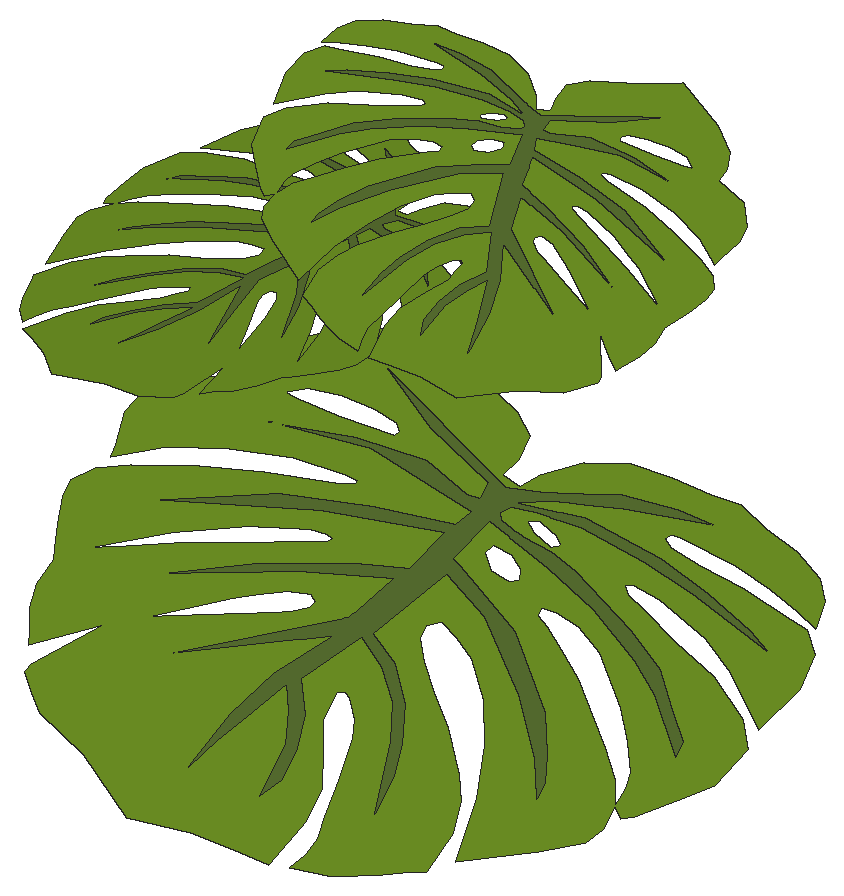
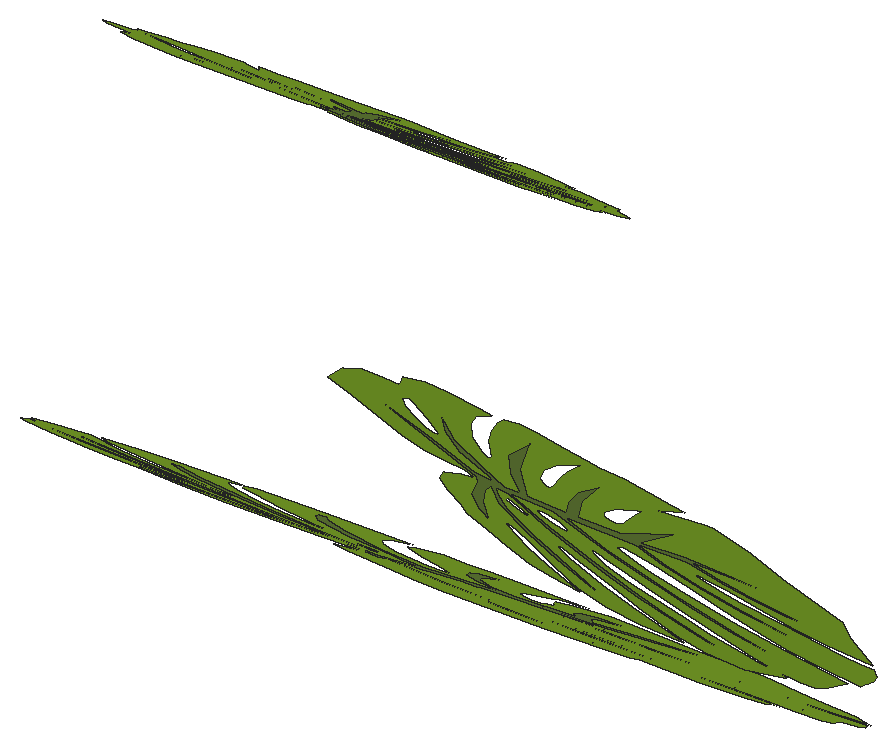
# SketchUp Ruby script. Lengths in inches.
U = 1.inch
M = Sketchup.active_model
def pt(a) = Geom::Point3d.new(a.map { |v| v * U })
def face(e, loops, mat)
  f = e.add_face(loops[0].map { |a| pt(a) })
  loops[1..].each { |l| e.add_face(l.map { |a| pt(a) }).erase! }
  f.material = f.back_material = mat if mat
  f
end
# faces: each face lists its corners as indices into pts; further lists are holes
def faces(e, pts, list, mat = nil) = list.each { |f| face(e, (f[0].is_a?(Array) ? f : [f]).map { |l| l.map { |i| pts[i] } }, mat) }
# xy, xz, yz: faces in a plane at the given z, y or x. An outline is a flat list of corners, or four numbers for a rectangle; further outlines are holes
def ring(l) = l.size == 4 ? [[l[0], l[1]], [l[2], l[1]], [l[2], l[3]], [l[0], l[3]]] : l.each_slice(2).to_a
def flat(e, list, mat, &to3) = list.each { |f| face(e, (f[0].is_a?(Array) ? f : [f]).map { |l| ring(l).map { |u, v| to3.(u, v) } }, mat) }
def xy(e, z, list, mat = nil) = flat(e, list, mat) { |x, y| [x, y, z] }
def xz(e, y, list, mat = nil) = flat(e, list, mat) { |x, z| [x, y, z] }
def yz(e, x, list, mat = nil) = flat(e, list, mat) { |y, z| [x, y, z] }
def lines(e, pts, list) = list.each { |a, b| e.add_line(pt(pts[a]), pt(pts[b])) }
# prism: a flat outline (further loops are holes) pulled along v
def prism(e, loops, v, mat = nil)
  f = face(e, loops, mat); d = Geom::Vector3d.new(v.map { |x| x * U })
  f.pushpull(f.normal.samedirection?(d) ? d.length : -d.length)
end
def box(e, o, s, mat = nil) = prism(e, [[o, [o[0] + s[0], o[1], o[2]], [o[0] + s[0], o[1] + s[1], o[2]], [o[0], o[1] + s[1], o[2]]]], [0, 0, s[2]], mat)
def at(x, y, z, deg = 0) = Geom::Transformation.translation(pt([x, y, z])) * Geom::Transformation.rotation(ORIGIN, Z_AXIS, deg.degrees)
def axes(o, x, y, z) = Geom::Transformation.new([*x, 0, *y, 0, *z, 0, *pt(o).to_a, 1])
def part(name) = M.definitions.add(name)
# library, detail: a bought-in or finely detailed component or shape, given as its bounding box
def library(name, o, s) = part(name).tap { |d| box(d.entities, o, s) }
def detail(e, o, s) = box(e.add_group.entities, o, s)
def put(e, d, t, mat = nil) = e.add_instance(d, t).tap { |i| i.material = mat if mat }
def group(e, t, mat = nil) = e.add_group.tap { |g| g.transformation = t; g.material = mat if mat }.entities
root = M.entities
M.materials.add("[0059_DarkOliveGreen]").color = [85, 107, 47]
M.materials.add("[0061_OliveDrab]").color = [107, 142, 35]
p = [[188.129,149.193,18.099],[188.867,149.058,18.014],[189.298,149.585,18.348],[190.36,150.31,18.808],[191.818,150.755,19.091],[193.373,150.829,19.137],
  [194.933,150.763,19.096],[196.031,150.815,19.129],[197.325,150.449,18.897],[198.752,150.179,18.725],[199.994,149.73,18.44],[200.614,149.188,18.096],
  [200.915,148.399,17.595],[199.983,148.646,17.752],[198.718,148.953,17.947],[197.142,149.21,18.11],[194.901,149.364,18.208],[194.528,149.346,18.197],
  [194.422,149.173,18.087],[194.792,149.025,17.992],[196.049,148.844,17.878],[197.794,148.7,17.786],[199.955,148.392,17.591],[200.649,148.277,17.518],
  [201.39,147.705,17.155],[201.656,146.671,16.499],[201.213,145.244,15.593],[199.186,146.416,16.337],[197.722,147.038,16.732],[195.507,147.571,17.07],
  [194.395,147.678,17.138],[194.138,147.574,17.072],[194.419,147.371,16.943],[195.175,147.16,16.809],[196.834,146.638,16.477],[198.753,146.128,16.154],
  [200.526,145.311,15.636],[201.296,144.606,15.188],[201.01,143.35,14.391],[200.17,142.585,13.905],[199.179,141.75,13.375],[198.796,141.571,13.262],
  [198.359,141.816,13.417],[198.34,142.391,13.782],[198.164,142.833,14.063],[197.452,143.604,14.552],[196.535,144.398,15.056],[194.732,145.61,15.825],
  [193.58,146.062,16.112],[192.594,146.201,16.2],[192.047,146.175,16.184],[192.087,145.93,16.028],[192.577,145.743,15.91],[193.472,145.3,15.629],
  [194.609,144.73,15.267],[195.942,143.84,14.702],[196.825,143.226,14.3125],[197.843,142.494,13.848],[198.477,141.088,12.955],[198.226,140.6,12.646],
  [196.938,139.896,12.199],[194.606,138.8,11.503],[193.981,140.617,12.657],[193.129,142.056,13.57],[192.137,143.23,14.315],[190.932,144.16,14.905],
  [190.019,144.561,15.159],[189.248,144.796,15.308],[188.854,144.543,15.148],[188.918,144.151,14.899],[189.522,143.599,14.549],[190.445,142.922,14.119],
  [191.601,142.158,13.635],[192.928,141.049,12.931],[193.535,140.393,12.514],[193.953,139.485,11.938],[193.917,138.258,11.159],[193.201,137.991,10.99],
  [192.644,137.733,10.826],[191.891,137.439,10.64],[190.959,137.164,10.465],[189.647,136.965,10.339],[189.848,137.459,10.653],[189.903,138.002,10.997],
  [189.65,138.637,11.4],[189.357,139.697,12.073],[188.928,140.921,12.85],[188.577,141.433,13.174],[188.004,141.944,13.499],[187.687,142.048,13.564],
  [187.478,141.93,13.49],[187.541,141.541,13.243],[187.618,141.066,12.941],[188.221,140.343,12.483],[189.007,139.283,11.81],[189.164,138.318,11.197],
  [188.938,136.839,10.259],[187.796,136.88,10.285],[185.892,136.872,10.28],[183.578,136.626,10.124],[180.962,137.808,10.874],[178.746,138.425,11.265],
  [178.105,138.881,11.555],[177.463,139.337,11.844],[177.507,139.613,12.019],[178.941,141.333,13.111],[177.775,140.577,12.631],[177.012,140.075,12.3125],
  [176.793,140.418,12.53],[176.307,141.026,12.916],[176.024,141.733,13.365],[176.039,142.501,13.852],[175.829,142.83,14.061],[175.425,143.481,14.474],
  [175.025,144.212,14.938],[174.931,144.734,15.269],[175.457,145.287,15.62],[176.472,145.703,15.884],[178.588,146.355,16.298],[180.695,146.882,16.633],
  [183.311,147.344,16.926],[183.782,147.484,17.014],[183.766,147.585,17.079],[183.287,147.633,17.109],[181.351,147.541,17.051],[179.186,147.123,16.786],
  [177.216,146.524,16.405],[175.678,145.718,15.894],[175.621,146.07,16.117],[175.211,146.999,16.707],[175.365,147.705,17.155],[176.295,148.579,17.709],
  [178.131,149.062,18.016],[178.046,149.587,18.349],[178.464,150.324,18.817],[179.9,151.18,19.36],[182.852,152.287,20.0625],[183.878,151.906,19.821],
  [185.497,151.464,19.541],[187.227,150.962,19.222],[188.163,150.469,18.909],[188.28,149.748,18.451],[186.321,144.017,14.814],[181.293,141.142,12.99],
  [186.24,143.358,14.396],[185.177,141.829,13.426],[184.672,140.327,12.472],[184.468,138.685,11.431],[184.456,138.537,11.336],[184.807,139.528,11.965],
  [185.147,140.273,12.438],[185.754,141.671,13.326],[186.359,140.997,12.898],[186.98,140.081,12.316],[187.232,138.529,11.331],[187.557,139.162,11.733],
  [187.407,140.089,12.321],[186.938,141.057,12.936],[186.087,141.953,13.504],[187.106,143.621,14.563],[188.335,143.066,14.211],[189.379,142.273,13.708],
  [190.165,141.23,13.045],[191.141,139.208,11.762],[190.956,140.348,12.486],[190.562,141.259,13.064],[189.802,142.331,13.745],[188.691,143.264,14.336],
  [187.386,143.8,14.676],[188.417,146.099,16.136],[190.482,145.372,15.674],[193.14,143.709,14.619],[194.924,142.243,13.688],[195.809,141.238,13.05],
  [195.735,141.694,13.34],[195.208,142.46,13.826],[194.277,143.523,14.501],[191.711,145.279,15.615],[190.098,145.909,16.015],[188.343,146.554,16.424],
  [188.687,147.865,17.256],[191.387,147.275,16.882],[193.696,146.646,16.483],[195.989,145.748,15.913],[197.288,145.093,15.497],[199.197,143.709,14.619],
  [199.125,144.153,14.901],[198.127,144.865,15.353],[196.931,145.765,15.924],[195.251,146.495,16.387],[192.3,147.451,16.993],[191.169,147.717,17.162],
  [189.991,147.814,17.224],[189.006,148.021,17.355],[188.827,148.205,17.472],[189.074,148.436,17.619],[189.921,148.55,17.691],[191.639,148.63,17.742],
  [194.227,148.373,17.579],[196.396,148.036,17.365],[199.833,147.347,16.928],[198.913,147.683,17.141],[196.86,148.225,17.485],[194.69,148.65,17.754],
  [191.522,148.919,17.925],[189.167,148.628,17.741],[190.269,149.024,17.992],[192.528,149.564,18.335],[195.591,150.03,18.63],[194.197,150.061,18.65],
  [192.205,149.877,18.534],[189.719,149.184,18.094],[188.455,148.922,17.927],[182.115,150.875,19.167],[184.903,149.66,18.396],[187.812,148.843,17.877],
  [187.888,148.371,17.578],[187.406,148.349,17.563],[185.477,148.816,17.86],[182.827,148.691,17.781],[179.841,148.194,17.465],[183.537,148.534,17.681],
  [186.02,148.188,17.462],[187.893,147.932,17.299],[187.683,147.459,16.999],[184.743,147.095,16.768],[181.598,146.492,16.385],[177.819,145.024,15.453],
  [183.264,146.4375,16.351],[187.487,147.13,16.79],[187.168,145.88,15.996],[185.391,145.463,15.732],[182.37,144.471,15.102],[179.481,143.175,14.28],
  [183.852,144.676,15.232],[186.868,145.42,15.705],[181.318,145.322,15.642],[179.931,144.754,15.282],[179.158,144.4375,15.081],[176.818,143.148,14.263],
  [177.739,143.491,14.48],[179.664,144.237,14.954],[181.6,144.884,15.365],[183.364,145.465,15.733],[184.099,145.711,15.889],[184.188,145.851,15.978],
  [183.917,145.913,16.018],[183.288,145.862,15.985],[183.102,143.689,14.606],[182.702,143.504,14.489],[182.317,143.327,14.376],[180.069,141.98,13.522],
  [181.913,142.642,13.942],[183.894,143.363,14.399],[184.397,143.538,14.51],[184.888,143.847,14.706],[184.964,144.066,14.845],[184.652,144.207,14.935],
  [183.888,144.05,14.835],[182.142,149.616,18.368],[181.478,149.63,18.376],[180.354,149.474,18.277],[179.71,149.129,18.059],[180.136,149.073,18.023],
  [181.896,149.053,18.011],[184.003,149.103,18.042],[184.069,149.259,18.141],[183.778,149.465,18.272],[182.806,149.603,18.359],[189.158,147.003,16.709],
  [189.695,146.619,16.466],[190.486,146.503,16.392],[190.797,146.639,16.478],[190.6,146.975,16.692],[190.022,147.242,16.861],[189.288,147.297,16.896],
  [190.742,148.251,17.501],[190.201,148.378,17.582],[189.807,148.252,17.502],[190.259,148.022,17.356],[191.078,147.823,17.23],[191.374,147.974,17.325],
  [190.964,148.199,17.468],[186.512,151.899,25.1],[187.3,151.802,25.26],[187.777,150.495,24.796],[187.751,149.711,24.4375],[187.345,149.255,24.129],
  [186.879,149.033,23.909],[187.343,148.316,23.706],[187.066,147.659,23.34],[186.5625,147.289,23.045],[185.615,146.965,22.655],[185.303,146.816,22.508],
  [185.241,147.604,22.846],[184.809,148.411,23.097],[184.139,149.185,23.272],[183.31,149.746,23.31],[183.047,149.852,23.29],[182.957,149.809,23.248],
  [183.064,149.618,23.189],[183.909,148.702,22.996],[184.463,147.892,22.775],[184.92,147.021,22.502],[185.055,146.556,22.328],[184.85,146.157,22.096],
  [184.382,145.938,21.877],[183.6,145.704,21.571],[182.882,145.509,21.299],[182.516,145.411,21.16],[181.898,145.049,20.839],[181.191,144.795,20.543],
  [180.469,144.641,20.288],[180.088,144.539,20.144],[180.141,144.978,20.355],[180.211,145.643,20.671],[179.48,144.456,19.951],[179.277,144.316,19.835],
  [178.606,144.275,19.644],[177.936,144.234,19.453],[176.4,144.538,19.195],[174.217,144.687,18.7],[173.337,145.421,18.803],[172.455,145.935,18.806],
  [171.889,146.221,18.789],[172.987,146.972,19.408],[173.846,147.38,19.813],[175.075,147.665,20.257],[175.945,147.841,20.559],[176.367,148.042,20.759],
  [176.713,148.206,20.921],[176.711,148.317,20.971],[176.479,148.354,20.927],[175.796,148.269,20.713],[175.216,148.124,20.499],[174.02,147.667,19.986],
  [173.02,147.251,19.542],[172.385,147.022,19.276],[171.969,146.754,19.049],[171.661,146.47,18.842],[171.21,146.914,18.925],[171,147.292,19.041],
  [170.887,147.63,19.163],[170.836,147.9,19.271],[170.72,148.216,19.383],[171.702,148.798,19.897],[172.636,149.11,20.278],[173.453,149.254,20.552],
  [174.975,149.416,21.017],[176.135,149.463,21.337],[177.117,149.532,21.621],[177.849,149.628,21.852],[178.197,149.794,22.016],[178.219,150.018,22.122],
  [177.668,150.114,22.023],[176.916,150.172,21.855],[175.597,150.06,21.466],[174.179,149.778,20.974],[172.61,149.334,20.371],[170.839,148.653,19.61],
  [170.643,149.789,20.069],[170.615,150.463,20.364],[170.894,150.757,20.569],[171.542,151.065,20.874],[172.335,151.244,21.158],[173.406,151.313,21.464],
  [174.317,151.363,21.722],[175.663,151.422,22.094],[176.658,151.384,22.333],[177.437,151.351,22.519],[177.817,151.307,22.597],[178.035,151.411,22.7],
  [177.801,151.569,22.71],[177.228,151.768,22.652],[176.322,151.865,22.463],[174.495,151.782,21.955],[173.42,151.657,21.622],[172.461,151.488,21.3],
  [172.019,151.329,21.115],[171.139,151.068,20.771],[171.106,151.254,20.846],[171.323,151.909,21.196],[171.553,152.491,21.516],[172.442,153.154,22.042],
  [173.375,153.277,22.338],[174.867,153.183,22.68],[176.178,152.907,22.893],[177.377,152.707,23.112],[177.902,152.603,23.201],[178.198,152.623,23.285],
  [178.163,152.74,23.329],[177.556,152.988,23.284],[176.089,153.332,23.061],[174.9,153.434,22.801],[173,153.429,22.31],[173.955,154.214,22.907],
  [174.92,154.625,23.341],[175.731,154.693,23.58],[176.149,154.561,23.628],[177.408,154.127,23.757],[178.339,153.727,23.818],[179.073,153.475,23.893],
  [179.367,153.445,23.955],[179.458,153.554,24.028],[179.298,153.663,24.035],[178.127,154.19,23.971],[177.183,154.492,23.863],[176.343,154.688,23.735],
  [175.706,154.822,23.631],[176.489,155.109,23.962],[177.22,155.196,24.189],[178.165,155.074,24.377],[179.05,154.818,24.49],[179.952,154.642,24.643],
  [180.422,154.324,24.621],[181.203,153.937,24.649],[181.869,153.487,24.618],[182.187,152.888,24.431],[182.093,152.266,24.128],[181.866,151.905,23.907],
  [182.319,151.77,23.964],[182.701,152.069,24.196],[183.342,152.375,24.498],[184.18,152.354,24.704],[185.396,152.126,24.915],[184.205,151.125,24.159],
  [186.495,150.946,24.668],[185.024,151.2,24.404],[181.947,151.731,23.85],[181.571,152.191,23.96],[180.975,153.18,24.25],[180.194,153.799,24.327],
  [179.518,154.158,24.314],[180.569,153.121,24.119],[181.183,152.264,23.893],[181.376,151.784,23.727],[180.513,152.55,23.849],[178.815,153.273,23.736],
  [177.457,153.655,23.558],[176.058,153.952,23.331],[175.355,154.041,23.19],[177.52,153.443,23.479],[178.807,153.02,23.62],[180.224,152.447,23.728],
  [180.96,151.95,23.694],[181.263,151.67,23.647],[181.19,151.496,23.55],[180.956,151.458,23.473],[180.329,151.625,23.386],[179.7,151.895,23.345],
  [178.955,152.073,23.234],[176.801,152.417,22.834],[175.422,152.526,22.528],[174.132,152.427,22.151],[173.087,152.361,21.853],[172.692,152.173,21.666],
  [174.708,152.308,22.246],[175.848,152.266,22.521],[177.649,152.072,22.897],[179.239,151.747,23.16],[180.979,151.3,23.407],[180.072,150.596,22.858],
  [178.729,150.765,22.588],[177.463,150.902,22.324],[174.837,150.77,21.589],[173.537,150.523,21.144],[172.668,150.306,20.823],[172.262,150.113,20.631],
  [173.493,150.345,21.053],[175.518,150.552,21.667],[178.112,150.617,22.363],[179.667,150.403,22.668],[178.278,149.054,21.705],[177.232,149.154,21.48],
  [175.955,149.016,21.09],[174.728,148.718,20.64],[173.802,148.399,20.259],[172.788,147.916,19.781],[174.889,148.599,20.628],[176.105,148.875,21.065],
  [177.238,148.966,21.397],[178.263,148.896,21.63],[177.381,147.845,20.931],[176.254,147.654,20.556],[175.248,147.328,20.15],[174.424,146.936,19.762],
  [174.06,146.553,19.497],[175.441,147.21,20.147],[176.476,147.471,20.531],[177.308,147.624,20.813],[176.453,146.809,20.227],[176.005,146.37,19.915],
  [175.362,145.814,19.5],[175.478,145.886,19.5625],[176.718,146.707,20.25],[177.705,147.544,20.879],[178.453,148.542,21.52],[178.958,146.183,20.591],
  [178.952,148.871,21.796],[179.838,149.672,22.383],[180.64,148.517,22.072],[181.459,146.647,21.443],[181.164,148.025,21.986],[180.562,149.296,22.401],
  [180.072,149.967,22.576],[180.941,150.635,23.1],[182.348,149.182,22.81],[183.739,147.065,22.217],[183.169,148.762,22.832],[182.193,149.885,23.085],
  [181.117,150.842,23.237],[181.404,151.119,23.435],[182.486,150.737,23.543],[183.927,150.234,23.688],[185.375,149.085,23.545],[184.385,150.117,23.753],
  [183.25,150.884,23.806],[181.97,151.183,23.61],[181.763,151.322,23.619],[182.183,151.522,23.817],[182.348,148.141,22.342],[181.868,148.92,22.568],
  [181.616,149.112,22.59],[181.439,149.156,22.564],[181.367,149.066,22.505],[181.51,148.755,22.402],[181.86,148.012,22.159],[182.237,147.192,21.888],
  [182.528,146.328,21.575],[182.679,145.922,21.432],[182.637,147.15,21.972],[180.114,148.235,21.809],[179.885,148.513,21.875],[179.625,148.53,21.816],
  [179.482,148.408,21.724],[179.459,148.132,21.595],[179.552,147.916,21.522],[179.89,147.049,21.22],[180.212,146.247,20.942],[180.259,147.477,21.507],
  [185.779,150.194,24.147],[185.137,150.537,24.135],[184.571,150.732,24.077],[184.268,150.714,23.991],[184.172,150.624,23.926],[185.115,150.037,23.905],
  [185.953,149.575,23.914],[186.197,149.487,23.937],[186.176,149.82,24.081],[179.849,151.366,23.146],[179.362,151.396,23.035],[178.996,151.292,22.894],
  [179.03,151.146,22.837],[179.494,150.988,22.885],[180.057,151.023,23.046],[180.236,151.196,23.169],[180.69,151.944,23.622],[180.1875,152.065,23.547],
  [179.813,152.07,23.453],[179.829,151.92,23.39],[180.373,151.794,23.473],[180.77,151.78,23.569],[190.337,148.724,31.73],[189.85,148.635,31.674],
  [189.565,148.982,31.894],[188.864,149.461,32.198],[187.902,149.755,32.385],[186.876,149.803,32.415],[185.846,149.76,32.388],[185.122,149.794,32.41],
  [184.267,149.553,32.256],[183.326,149.375,32.143],[182.506,149.078,31.955],[182.097,148.72,31.728],[181.898,148.2,31.398],[182.513,148.363,31.501],
  [183.348,148.565,31.63],[184.388,148.735,31.737],[185.867,148.837,31.802],[186.114,148.825,31.794],[186.184,148.711,31.722],[185.939,148.613,31.66],
  [185.11,148.494,31.584],[183.958,148.398,31.524],[182.532,148.195,31.395],[182.074,148.119,31.346],[181.584,147.742,31.107],[181.409,147.06,30.674],
  [181.702,146.117,30.076],[183.039,146.891,30.567],[184.005,147.302,30.828],[185.467,147.653,31.051],[186.201,147.724,31.096],[186.371,147.655,31.052],
  [186.186,147.521,30.967],[185.687,147.382,30.878],[184.592,147.037,30.66],[183.325,146.701,30.446],[182.155,146.162,30.104],[181.647,145.696,29.809],
  [181.835,144.867,29.283],[182.39,144.362,28.962],[183.044,143.811,28.613],[183.297,143.693,28.538],[183.585,143.855,28.64],[183.598,144.234,28.881],
  [183.713,144.526,29.066],[184.184,145.035,29.389],[184.789,145.559,29.722],[185.979,146.359,30.229],[186.739,146.657,30.419],[187.39,146.749,30.477],
  [187.751,146.732,30.466],[187.724,146.57,30.363],[187.402,146.447,30.285],[186.81,146.155,30.1],[186.06,145.778,29.861],[185.18,145.191,29.488],
  [184.597,144.786,29.231],[183.926,144.302,28.924],[183.507,143.374,28.335],[183.673,143.053,28.131],[184.523,142.588,27.836],[186.062,141.864,27.377],
  [186.474,143.064,28.138],[187.037,144.014,28.741],[187.692,144.788,29.233],[188.487,145.402,29.622],[189.089,145.666,29.79],[189.598,145.822,29.888],
  [189.858,145.655,29.782],[189.816,145.396,29.618],[189.418,145.032,29.387],[188.808,144.585,29.103],[188.046,144.081,28.784],[187.17,143.349,28.319],
  [186.769,142.916,28.044],[186.493,142.316,27.664],[186.517,141.507,27.15],[186.989,141.33,27.038],[187.357,141.16,26.93],[187.854,140.966,26.807],
  [188.469,140.784,26.691],[189.335,140.653,26.608],[189.202,140.98,26.815],[189.166,141.338,27.043],[189.333,141.757,27.309],[189.527,142.457,27.753],
  [189.81,143.264,28.265],[190.041,143.602,28.48],[190.419,143.94,28.694],[190.628,144.008,28.737],[190.767,143.93,28.688],[190.725,143.674,28.525],
  [190.674,143.36,28.326],[190.276,142.883,28.023],[189.757,142.183,27.579],[189.654,141.546,27.175],[189.803,140.57,26.555],[190.557,140.597,26.573],
  [191.813,140.592,26.569],[193.34,140.43,26.466],[195.067,141.209,26.961],[196.53,141.617,27.22],[196.953,141.918,27.411],[197.376,142.219,27.602],
  [197.347,142.401,27.717],[196.401,143.536,28.438],[197.171,143.038,28.121],[197.674,142.706,27.911],[197.819,142.932,28.054],[198.139,143.334,28.309],
  [198.326,143.8,28.605],[198.316,144.307,28.927],[198.455,144.525,29.065],[198.721,144.954,29.338],[198.986,145.436,29.644],[199.048,145.781,29.862],
  [198.701,146.146,30.094],[198.031,146.42,30.268],[196.634,146.851,30.542],[195.244,147.199,30.762],[193.517,147.503,30.956],[193.206,147.596,31.014],
  [193.217,147.663,31.057],[193.533,147.694,31.077],[194.81,147.634,31.038],[196.239,147.358,30.863],[197.54,146.962,30.612],[198.555,146.43,30.275],
  [198.592,146.662,30.422],[198.862,147.276,30.811],[198.761,147.742,31.107],[198.147,148.318,31.473],[196.935,148.637,31.675],[196.991,148.984,31.895],
  [196.716,149.471,32.204],[195.768,150.035,32.5625],[193.819,150.766,33.026],[193.143,150.514,32.867],[192.074,150.223,32.682],[190.932,149.891,32.471],
  [190.315,149.566,32.265],[190.237,149.09,31.963],[191.53,145.308,29.562],[194.849,143.41,28.358],[191.583,144.873,29.286],[192.285,143.864,28.646],
  [192.619,142.872,28.016],[192.753,141.789,27.329],[192.761,141.691,27.267],[192.529,142.345,27.682],[192.305,142.837,27.994],[191.905,143.76,28.58],
  [191.505,143.314,28.297],[191.095,142.71,27.913],[190.929,141.685,27.263],[190.714,142.104,27.529],[190.814,142.715,27.917],[191.123,143.354,28.322],
  [191.685,143.945,28.698],[191.012,145.046,29.396],[190.201,144.68,29.164],[189.512,144.157,28.832],[188.993,143.468,28.395],[188.349,142.134,27.548],
  [188.471,142.886,28.025],[188.731,143.487,28.407],[189.233,144.195,28.856],[189.966,144.81,29.247],[190.827,145.164,29.471],[190.147,146.682,30.434],
  [188.784,146.202,30.13],[187.029,145.104,29.433],[185.852,144.137,28.819],[185.268,143.473,28.398],[185.317,143.775,28.589],[185.665,144.28,28.91],
  [186.279,144.982,29.355],[187.973,146.141,30.091],[189.037,146.556,30.355],[190.196,146.982,30.625],[189.969,147.847,31.174],[188.186,147.458,30.927],
  [186.663,147.043,30.663],[185.149,146.45,30.287],[184.292,146.018,30.013],[183.032,145.104,29.433],[183.08,145.397,29.619],[183.738,145.868,29.918],
  [184.527,146.462,30.294],[185.637,146.943,30.6],[187.584,147.574,31],[188.33,147.749,31.112],[189.108,147.814,31.153],[189.758,147.95,31.239],
  [189.876,148.072,31.316],[189.713,148.224,31.413],[189.154,148.299,31.461],[188.02,148.353,31.495],[186.312,148.183,31.387],[184.881,147.96,31.246],
  [182.612,147.505,30.957],[183.219,147.727,31.098],[184.575,148.085,31.325],[186.007,148.365,31.503],[188.097,148.543,31.615],[189.652,148.351,31.494],
  [188.924,148.612,31.659],[187.433,148.969,31.886],[185.412,149.276,32.081],[186.332,149.297,32.094],[187.647,149.176,32.017],[189.288,148.718,31.726],
  [190.122,148.545,31.617],[194.306,149.834,32.435],[192.466,149.032,31.926],[190.546,148.493,31.583],[190.496,148.181,31.386],[190.814,148.166,31.376],
  [192.087,148.475,31.572],[193.836,148.392,31.52],[195.807,148.064,31.312],[193.368,148.289,31.454],[191.729,148.061,31.309],[190.492,147.892,31.202],
  [190.631,147.579,31.004],[192.572,147.339,30.852],[194.647,146.941,30.599],[197.142,145.972,29.984],[193.548,146.905,30.576],[190.761,147.362,30.866],
  [190.971,146.537,30.342],[192.144,146.262,30.168],[194.138,145.607,29.752],[196.045,144.752,29.21],[193.16,145.742,29.838],[191.169,146.234,30.15],
  [194.832,146.169,30.109],[195.748,145.794,29.871],[196.258,145.585,29.738],[197.802,144.734,29.198],[197.194,144.96,29.342],[195.924,145.453,29.654],
  [194.646,145.88,29.925],[193.482,146.263,30.169],[192.997,146.425,30.272],[192.938,146.518,30.33],[193.117,146.559,30.356],[193.532,146.525,30.335],
  [193.655,145.091,29.425],[193.919,144.969,29.347],[194.173,144.852,29.273],[195.656,143.963,28.709],[194.439,144.4,28.986],[193.132,144.876,29.288],
  [192.8,144.991,29.361],[192.476,145.195,29.491],[192.426,145.34,29.583],[192.632,145.433,29.642],[193.136,145.33,29.576],[194.288,149.003,31.907],
  [194.727,149.012,31.913],[195.468,148.909,31.848],[195.893,148.682,31.704],[195.612,148.645,31.68],[194.451,148.632,31.672],[193.06,148.665,31.693],
  [193.016,148.767,31.758],[193.209,148.903,31.844],[193.85,148.994,31.902],[189.658,147.278,30.813],[189.303,147.025,30.652],[188.781,146.948,30.603],
  [188.576,147.038,30.66],[188.706,147.26,30.801],[189.088,147.436,30.913],[189.572,147.472,30.936],[188.612,148.102,31.336],[188.97,148.186,31.389],
  [189.229,148.103,31.336],[188.931,147.951,31.24],[188.39,147.82,31.156],[188.195,147.919,31.219],[188.466,148.067,31.314],[190.605,146.973,16.69],
  [188.703,147.258,30.8]]
faces(root,p,[[[0,1,2,3,4,5,6,7,8,9,10,11,12,13,14,15,16,17,18,19,20,21,22,23,24,25,26,27,28,29,30,31,32,33,34,35,36,37,38,39,40,41,42,43,44,45,46,47,48,49,50,51,52,53,54,55,56,57,42,58,59,60,61,62,63,64,65,66,67,68,69,70,71,72,73,74,75,76,77,78,79,80,81,82,83,84,85,86,87,88,89,90,91,92,93,94,95,96,97,98,99,100,101,102,103,104,105,106,107,108,109,110,111,112,113,114,115,116,117,118,119,120,121,122,123,124,125,126,127,128,129,130,131,132,133,134,135,136,137,138,139,140,141],[142,143,144,145,146,147,148,149,150,151,152,153,154,155,156,157,158,159,160,161,162,163,164,165,166,167,168,169,170,171,172,173,174,175,176,177,178,179,180,181,182,183,184,185,186,187,188,189,190,191,192,193,194,195,196,197,198,199,200,201,202,203,204,205,206,207,208,209,210,211,212,213,214,215,216,217,218,219,220,221,222,223,224,225,226,227,228,229,230,231,232,233,234,235],[236,237,238,239,240,241,242,243,244,245,246,247],[248,249,250,251,252,253,254,255,256,257,258],[259,260,261,262,263,264,265,266,267,268],[269,270,271,272,273,274,275],[276,277,278,279,280,281,282]],[[283,284,285,286,287,288,289,290,291,292,293,294,295,296,297,298,299,300,301,302,303,304,305,306,307,308,309,310,311,312,313,314,315,316,317,318,319,320,321,322,323,324,325,326,327,328,329,330,331,332,333,334,335,336,337,338,339,340,341,342,343,344,345,346,347,348,349,350,351,352,353,354,355,356,357,358,359,360,361,362,363,364,365,366,367,368,369,370,371,372,373,374,375,376,377,378,363,379,380,381,382,383,384,385,386,387,388,389,390,391,392,393,394,395,396,397,398,399,400,401,402,403,404,405,406,407,408,409,410,411,412,413,414,415,416,417,418,419,420,421,422,423,424],[425,426,427,428,429,430,431,432,433,434,435,436,437,438,439,440,441,442,443,444,445,446,447,448,449,450,451,452,453,454,455,456,457,458,459,460,461,462,463,464,465,466,467,468,469,470,471,472,473,474,475,476,477,478,479,480,481,482,483,484,485,486,487,488,489,490,491,492,493,494,495,496,497,498,499,500,501,502,503,504,505,506,507,508,509,510,511,512,513,514,515,516,517,518,519],[520,521,522,523,524,525,526,527,528,529,530],[531,532,533,534,535,536,537,538,539],[540,541,542,543,544,545,546,547,548],[549,550,551,552,553,554,555],[556,557,558,559,560,561]],[[562,563,564,565,566,567,568,569,570,571,572,573,574,575,576,577,578,579,580,581,582,583,584,585,586,587,588,589,590,591,592,593,594,595,596,597,598,599,600,601,602,603,604,605,606,607,608,609,610,611,612,613,614,615,616,617,618,619,604,620,621,622,623,624,625,626,627,628,629,630,631,632,633,634,635,636,637,638,639,640,641,642,643,644,645,646,647,648,649,650,651,652,653,654,655,656,657,658,659,660,661,662,663,664,665,666,667,668,669,670,671,672,673,674,675,676,677,678,679,680,681,682,683,684,685,686,687,688,689,690,691,692,693,694,695,696,697,698,699,700,701,702,703],[704,705,706,707,708,709,710,711,712,713,714,715,716,717,718,719,720,721,722,723,724,725,726,727,728,729,730,731,732,733,734,735,736,737,738,739,740,741,742,743,744,745,746,747,748,749,750,751,752,753,754,755,756,757,758,759,760,761,762,763,764,765,766,767,768,769,770,771,772,773,774,775,776,777,778,779,780,781,782,783,784,785,786,787,788,789,790,791,792,793,794,795,796,797],[798,799,800,801,802,803,804,805,806,807,808,809],[810,811,812,813,814,815,816,817,818,819,820],[821,822,823,824,825,826,827,828,829,830],[831,832,833,834,835,836,837],[838,839,840,841,842,843,844]]],"[0061_OliveDrab]")
faces(root,p,[[143,142,235,234,233,232,231,230,229,228,227,226,225,224,223,222,221,220,219,218,217,216,215,214,213,212,211,210,209,208,207,206,205,204,203,202,201,200,199,198,197,196,195,194,193,192,191,190,189,188,187,186,185,184,183,182,181,180,179,178,177,176,175,174,173,172,171,170,169,168,167,166,165,164,163,162,161,160,159,158,157,156,155,154,153,152,151,150,149,148,147,146,145,144],[426,425,519,518,517,516,515,514,513,512,511,510,509,508,507,506,505,504,503,502,501,500,499,498,497,496,495,494,493,492,491,490,489,488,487,486,485,484,483,482,481,480,479,478,477,476,475,474,473,472,471,470,469,468,467,466,465,464,463,462,461,460,459,458,457,456,455,454,453,452,451,450,449,448,447,446,445,444,443,442,441,440,439,438,437,436,435,434,433,432,431,430,429,428,427],[705,704,797,796,795,794,793,792,791,790,789,788,787,786,785,784,783,782,781,780,779,778,777,776,775,774,773,772,771,770,769,768,767,766,765,764,763,762,761,760,759,758,757,756,755,754,753,752,751,750,749,748,747,746,745,744,743,742,741,740,739,738,737,736,735,734,733,732,731,730,729,728,727,726,725,724,723,722,721,720,719,718,717,716,715,714,713,712,711,710,709,708,707,706]],"[0059_DarkOliveGreen]")
lines(root,p,[[273,845],[835,846]])
